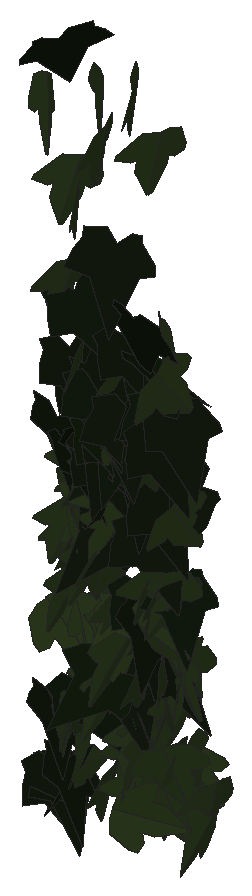
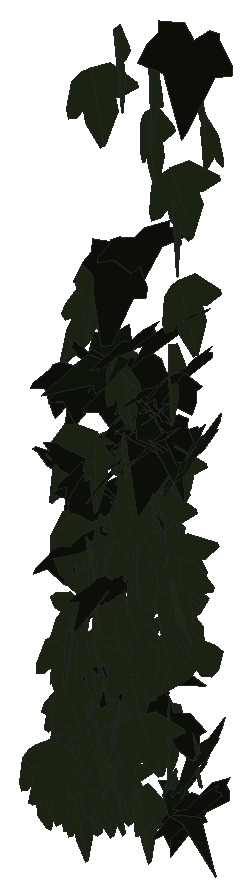
# SketchUp Ruby script. Lengths in inches.
U = 1.inch
M = Sketchup.active_model
def pt(a) = Geom::Point3d.new(a.map { |v| v * U })
def face(e, loops, mat)
  f = e.add_face(loops[0].map { |a| pt(a) })
  loops[1..].each { |l| e.add_face(l.map { |a| pt(a) }).erase! }
  f.material = f.back_material = mat if mat
  f
end
# faces: each face lists its corners as indices into pts; further lists are holes
def faces(e, pts, list, mat = nil) = list.each { |f| face(e, (f[0].is_a?(Array) ? f : [f]).map { |l| l.map { |i| pts[i] } }, mat) }
# xy, xz, yz: faces in a plane at the given z, y or x. An outline is a flat list of corners, or four numbers for a rectangle; further outlines are holes
def ring(l) = l.size == 4 ? [[l[0], l[1]], [l[2], l[1]], [l[2], l[3]], [l[0], l[3]]] : l.each_slice(2).to_a
def flat(e, list, mat, &to3) = list.each { |f| face(e, (f[0].is_a?(Array) ? f : [f]).map { |l| ring(l).map { |u, v| to3.(u, v) } }, mat) }
def xy(e, z, list, mat = nil) = flat(e, list, mat) { |x, y| [x, y, z] }
def xz(e, y, list, mat = nil) = flat(e, list, mat) { |x, z| [x, y, z] }
def yz(e, x, list, mat = nil) = flat(e, list, mat) { |y, z| [x, y, z] }
def lines(e, pts, list) = list.each { |a, b| e.add_line(pt(pts[a]), pt(pts[b])) }
# prism: a flat outline (further loops are holes) pulled along v
def prism(e, loops, v, mat = nil)
  f = face(e, loops, mat); d = Geom::Vector3d.new(v.map { |x| x * U })
  f.pushpull(f.normal.samedirection?(d) ? d.length : -d.length)
end
def box(e, o, s, mat = nil) = prism(e, [[o, [o[0] + s[0], o[1], o[2]], [o[0] + s[0], o[1] + s[1], o[2]], [o[0], o[1] + s[1], o[2]]]], [0, 0, s[2]], mat)
def at(x, y, z, deg = 0) = Geom::Transformation.translation(pt([x, y, z])) * Geom::Transformation.rotation(ORIGIN, Z_AXIS, deg.degrees)
def axes(o, x, y, z) = Geom::Transformation.new([*x, 0, *y, 0, *z, 0, *pt(o).to_a, 1])
def part(name) = M.definitions.add(name)
# library, detail: a bought-in or finely detailed component or shape, given as its bounding box
def library(name, o, s) = part(name).tap { |d| box(d.entities, o, s) }
def detail(e, o, s) = box(e.add_group.entities, o, s)
def put(e, d, t, mat = nil) = e.add_instance(d, t).tap { |i| i.material = mat if mat }
def group(e, t, mat = nil) = e.add_group.tap { |g| g.transformation = t; g.material = mat if mat }.entities
root = M.entities
M.materials.add("efeu1").color = [18, 25, 13]
M.materials.add("efeu2").color = [43, 57, 29]
c1 = part("ivyleaf_9")
p = [[1.54,2.16,1.25],[1.36,2.04,1.19],[-0.21,0.99,0.68],[-0.71,1.11,0.82],[-0.85,0.86,0.67],[-0.8,0.17,0.21],
  [-0.9,-0.01,0.1],[-0.67,-0.16,-0.02],[-0.08,-0.08,-0.05],[-0.03,-0.6,-0.4],[0.65,-0.88,-0.66],[0.83,-0.6,-0.49],
  [1.29,-0.42,-0.43],[1.8125,-0.07,-0.26],[1.21,0.44,0.15]]
faces(c1.entities,p,[[0,1,2,3,4,5,6,7,8,9,10,11,12,13,14]],"efeu1")
c2 = part("ivyleaf_10")
p = [[0,0.5,-0.03],[-0.0625,2.02,-0.43],[-0.19,2.01,-0.46],[-0.54,1.05,-0.29],[-0.52,0.625,-0.18],[-0.83,0.76,-0.28],
  [-1.16,0.64,-0.33],[-1.15,0.33,-0.24],[-0.77,-0.39,0.02],[-0.3,-0.51,0.16],[0.04,-0.48,0.23],[-0.02,2.01,-0.4375],
  [-0.06,2.01,-0.43],[0.04,-0.49,0.23],[0.67,-0.49,0.14],[1.38,0.36,-0.2],[1.375,0.51,-0.24],[0.81,0.65,-0.19],
  [0.62,0.59,-0.15],[0.6,1.09,-0.28],[0.5,1.23,-0.31]]
faces(c2.entities,p,[[0,1,2,3,4,5,6,7,8,9,10],[11,12,0,13,14,15,16,17,18,19,20]],"efeu2")
put(root,c1,axes([512.25,136.02,185.85],[0.17121,-0.66389,0.41643],[0.14297,-0.39264,-0.68474],[0.77053,0.22037,0.03452]))
put(root,c2,axes([512.8,136.1,191.76],[-0.23988,-0.65077,0.29698],[-0.05706,-0.29483,-0.69214],[0.71305,-0.24252,0.04452]))
put(root,c2,axes([512.39,135.42,204.18],[0.63102,-0.41173,0.31313],[0.32609,-0.06679,-0.74496],[0.40155,0.70127,0.11289]))
put(root,c2,axes([512.73,136.19,190.89],[0.29316,-0.70256,0.01967],[0.00631,-0.01868,-0.76127],[0.70281,0.29322,-0.00137]))
put(root,c1,axes([513.13,135.59,184.39],[-0.43077,0.62259,0.10496],[-0.07146,0.07817,-0.75695],[-0.62732,-0.43643,0.01415]))
put(root,c2,axes([512.82,136.26,191.31],[-0.52598,-0.52412,-0.07313],[0.07237,0.03089,-0.74197],[0.52422,-0.53014,0.02906]))
put(root,c2,axes([512.87,136.08,189.88],[0.00273,-0.64219,0.39214],[0.02346,-0.39188,-0.64193],[0.75209,0.01456,0.0186]))
put(root,c1,axes([512.58,135.55,184.57],[0.11322,-0.65761,-0.38062],[-0.08148,0.3721,-0.66712],[0.75544,0.1387,-0.01491]))
put(root,c1,axes([512.63,135.93,184.36],[0.09548,-0.75103,-0.16729],[-0.02977,0.16484,-0.75703],[0.76886,0.09965,-0.00854]))
put(root,c2,axes([513,135.64,199.0625],[-0.11608,-0.78207,0.08337],[-0.01662,-0.08182,-0.79062],[0.78632,-0.11718,-0.0044]))
put(root,c2,axes([512.55,135.68,188.94],[0.43104,0.49262,0.46939],[0.30894,0.35339,-0.65457],[-0.60626,0.53032,0.00017]))
put(root,c1,axes([512.62,135.67,194.54],[0.19979,-0.68286,0.34135],[0.14695,-0.31185,-0.70986],[0.74915,0.24328,0.04821]))
put(root,c2,axes([513.19,135.29,186.32],[0.52518,-0.53151,-0.21282],[-0.13994,0.16087,-0.74709],[0.55517,0.54335,0.01301]))
put(root,c1,axes([513.22,135,206.06],[0.26904,0.77907,-0.13785],[-0.0424,-0.1312,-0.82421],[-0.79003,0.27235,-0.00271]))
put(root,c2,axes([513.16,135.91,184.79],[0.16834,-0.33193,-0.63703],[0.04962,0.6581,-0.32979],[0.7166,0.0324,0.17249]))
put(root,c2,axes([513.35,136.875,186.88],[-0.5621,-0.38238,0.26694],[-0.08089,-0.33178,-0.6456],[0.45926,-0.52643,0.213]))
put(root,c2,axes([513.35,135.53,202.18],[-0.32855,-0.70465,0.21746],[-0.00138,-0.23747,-0.7716],[0.73744,-0.31439,0.09544]))
put(root,c2,axes([513.24,135.64,201.43],[0.46456,-0.6346,-0.16218],[0.02329,0.21472,-0.77343],[0.65459,0.44274,0.14262]))
put(root,c2,axes([513.84,135.73,191.36],[-0.22843,0.05655,0.74398],[-0.74006,-0.11613,-0.2184],[0.0949,-0.76954,0.08763]))
put(root,c2,axes([513.37,135.58,186.62],[0.19506,-0.62436,-0.44065],[-0.0684,0.43869,-0.65186],[0.76113,0.19943,0.05435]))
put(root,c2,axes([513.39,136.28,192.96],[-0.29712,-0.70174,0.08196],[-0.02507,-0.07839,-0.76201],[0.70607,-0.29808,0.00743]))
put(root,c2,axes([513.16,136.48,188.93],[0.30224,0.67377,0.01159],[0.00109,0.01222,-0.73844],[-0.67386,0.30222,0.00401]))
put(root,c1,axes([512.93,135.6875,184.65],[0.26823,-0.71704,0.18582],[0.04112,-0.18291,-0.76517],[0.73959,0.27022,-0.02485]))
put(root,c2,axes([513.28,136.06,192.25],[0.17181,0.63478,0.40598],[-0.04092,0.42365,-0.64508],[-0.75239,0.12191,0.12779]))
put(root,c2,axes([513.4,136.04,191.22],[-0.44298,0.6305,0.26282],[0.11574,-0.23944,0.76949],[0.67321,0.45604,0.04065]))
put(root,c2,axes([513.47,135.5,196.96],[0.28545,-0.66525,-0.30561],[-0.04253,0.3124,-0.71975],[0.73086,0.278,0.07748]))
put(root,c2,axes([513.48,135.84,193.11],[0.14567,-0.76213,-0.00746],[-0.00245,0.00712,-0.77593],[0.76217,0.14568,-0.00107]))
put(root,c1,axes([513.14,135.54,196.76],[0.19066,-0.74802,-0.1562],[-0.0054,0.15966,-0.77121],[0.76414,0.18776,0.03352]))
put(root,c1,axes([513.09,135.84,198.26],[0.2356,-0.67759,-0.31851],[0.08286,0.35545,-0.69489],[0.74412,0.17495,0.17822]))
put(root,c2,axes([513.7,135.63,193.89],[-0.52211,-0.50137,0.25286],[-0.09213,-0.2641,-0.71391],[0.55391,-0.51651,0.11959]))
put(root,c2,axes([513.66,135.96,190.96],[-0.11803,-0.65996,0.36858],[-0.02879,-0.36885,-0.66966],[0.75536,-0.11718,0.03207]))
put(root,c1,axes([513.2,135.33,194.15],[0.50606,-0.58909,0.01522],[0.00808,-0.01313,-0.77661],[0.58923,0.50612,-0.00243]))
put(root,c1,axes([513.2,135.91,186.97],[-0.13591,-0.25755,-0.75391],[0.55722,0.51589,-0.27669],[0.56941,-0.56632,0.09082]))
put(root,c2,axes([513.76,136.35,184.31],[0.17597,-0.72027,-0.09053],[-0.01826,0.08873,-0.74145],[0.72571,0.17688,0.0033]))
put(root,c1,axes([514.12,135.24,195.02],[-0.32198,0.72176,0.01967],[-0.00865,0.01767,-0.79032],[-0.72197,-0.32209,0.0007]))
put(root,c1,axes([513.93,135.43,194.88],[0.3543,0.74278,-0.06207],[-0.03684,-0.05119,-0.82287],[-0.74446,0.35603,0.01119]))
put(root,c2,axes([514.02,136.53,188.28],[-0.2659,-0.69247,0.08325],[-0.02154,-0.0809,-0.74171],[0.69712,-0.26662,0.00884]))
put(root,c2,axes([514.41,136.86,184.91],[-0.27999,0.21572,0.6234],[-0.58852,0.22425,-0.34193],[-0.298,-0.64555,0.08954]))
put(root,c2,axes([514.15,136.04,193.51],[-0.1752,-0.75203,0.11088],[-0.01439,-0.11049,-0.77209],[0.76002,-0.17545,0.01094]))
put(root,c2,axes([514.26,135.87,191.35],[-0.57986,-0.45419,0.14176],[-0.10103,-0.10084,-0.73637],[0.46494,-0.58835,0.01678]))
put(root,c2,axes([514.18,135.55,191.25],[0.08005,-0.75655,-0.10705],[-0.00412,0.1072,-0.76074],[0.76408,0.07984,0.00711]))
put(root,c2,axes([513.6875,135.08,193.375],[0.01712,-0.22317,0.76558],[0.45523,0.63146,0.17389],[-0.65474,0.43321,0.14093]))
put(root,c1,axes([513.7,135.53,196.51],[-0.13786,-0.34361,-0.6958],[0.46042,0.53265,-0.35426],[0.62467,-0.46843,0.10756]))
put(root,c2,axes([514.16,135.9,187.23],[-0.03601,-0.55699,0.49682],[0.10069,-0.49647,-0.54931],[0.73954,0.04047,0.09898]))
put(root,c1,axes([514.4,135.74,187.78],[-0.56306,-0.4476,0.28525],[-0.202,-0.20385,-0.7186],[0.49083,-0.59737,0.03149]))
put(root,c2,axes([514.21,136.24,189.62],[0.03679,-0.74511,0.13637],[0.03521,-0.1347,-0.74549],[0.75667,0.04249,0.02806]))
put(root,c2,axes([514.24,135.43,203.4375],[0.18275,-0.78477,-0.11098],[0.00147,0.11422,-0.80531],[0.79257,0.18073,0.02708]))
put(root,c1,axes([514.66,135.18,193.3],[-0.2741,0.59282,0.51746],[-0.22474,0.46615,-0.65309],[-0.75412,-0.3544,0.00655]))
put(root,c1,axes([514.03,136.02,194.24],[-0.08895,-0.74088,0.20839],[-0.01658,-0.20788,-0.74616],[0.76945,-0.09013,0.00801]))
put(root,c1,axes([513.95,135.58,194.28],[0.27097,-0.66444,-0.29611],[-0.02825,0.30614,-0.71279],[0.72689,0.25959,0.08268]))
put(root,c2,axes([514.28,135.29,204.91],[0.56963,-0.56149,-0.18704],[0.01429,0.27258,-0.77474],[0.59165,0.534,0.1988]))
put(root,c1,axes([514.59,135.61,192.25],[-0.81295,-0.15313,-0.03686],[0.03748,0.00013,-0.82722],[0.15298,-0.81379,0.0068]))
put(root,c1,axes([513.98,135.56,196.05],[0.12458,-0.77171,-0.14079],[0.10346,0.15748,-0.7716],[0.77759,0.10269,0.12522]))
put(root,c2,axes([514.37,136.06,194.59],[0.20582,-0.74294,0.04333],[0.05377,-0.03,-0.76968],[0.74226,0.20819,0.04374]))
put(root,c1,axes([514.67,136.08,194.47],[-0.7419,-0.19795,0.05758],[-0.0545,-0.01909,-0.76784],[0.19883,-0.74389,0.00438]))
put(root,c2,axes([514.4,135.78,191.11],[0.12669,-0.69615,-0.24596],[0.0853,0.26168,-0.69672],[0.73338,0.08983,0.12353]))
put(root,c2,axes([514.5,136.94,185.91],[0.21403,-0.68514,0.11083],[0.01362,-0.11181,-0.71751],[0.69391,0.21352,-0.0201]))
put(root,c2,axes([514.48,135.76,188.45],[0.00445,-0.57781,0.48339],[0.10521,-0.47819,-0.57256],[0.74597,0.07089,0.07787]))
put(root,c2,axes([514.57,136.14,196.52],[-0.01684,-0.77554,0.00348],[-0.00083,-0.00347,-0.77572],[0.77555,-0.01685,-0.00076]))
put(root,c2,axes([514.6,136.55,185.46],[-0.29293,-0.65264,0.18639],[0.00575,-0.20539,-0.71012],[0.67871,-0.27994,0.08646]))
put(root,c2,axes([514.67,135.66,192.41],[-0.24468,-0.60599,0.41848],[-0.06904,-0.42016,-0.64878],[0.7332,-0.24179,0.07857]))
put(root,c2,axes([514.35,135.8,188.2],[0.28379,0.33168,-0.70111],[0.34152,0.61686,0.43006],[0.69637,-0.4377,0.07481]))
put(root,c1,axes([514.24,135.66,194.93],[0.31041,-0.69709,-0.19095],[0.0485,0.22743,-0.75145],[0.72114,0.28476,0.13273]))
put(root,c1,axes([514.29,135.41,195.13],[0.22789,-0.68741,-0.30167],[0.02736,0.32266,-0.71457],[0.75019,0.19705,0.1177]))
put(root,c2,axes([514.55,136.49,185.25],[-0.17048,0.66531,-0.22893],[0.06062,-0.22079,-0.68679],[-0.70098,-0.1809,-0.00372]))
put(root,c1,axes([514.53,135.67,200.21],[-0.25262,-0.74161,-0.16443],[0.04273,0.15913,-0.78339],[0.75842,-0.25599,-0.01063]))
put(root,c1,axes([515.03,135.67,195.92],[-0.75708,0.20191,-0.12469],[0.11088,-0.06762,-0.7827],[-0.20981,-0.76429,0.03631]))
put(root,c2,axes([514.74,136.13,186.375],[-0.45154,0.56141,0.074],[-0.05217,0.05299,-0.72043],[-0.56386,-0.45448,0.0074]))
put(root,c2,axes([514.82,136.76,184.71],[-0.07405,-0.71007,0.10685],[-0.00795,-0.1066,-0.71392],[0.71802,-0.07441,0.00311]))
put(root,c2,axes([514.69,135.63,194.9],[0.05471,0.76286,-0.02279],[-0.00098,-0.02278,-0.76482],[-0.7632,0.05471,-0.00065]))
put(root,c1,axes([514.46,136.0625,197.37],[0.26223,-0.67127,-0.29909],[-0.00477,0.316,-0.71341],[0.73487,0.24158,0.10209]))
put(root,c1,axes([514.5625,136.08,187.79],[-0.26325,-0.56288,-0.47031],[0.22757,0.41236,-0.62089],[0.69731,-0.34707,0.02507]))
put(root,c2,axes([514.96,136.08,184.59],[-0.35461,-0.56352,0.25401],[-0.0609,-0.25957,-0.66086],[0.61512,-0.35056,0.081]))
put(root,c2,axes([514.85,136.18,186.51],[-0.50662,0.51359,0.07012],[-0.0453,0.05381,-0.72139],[-0.51637,-0.50861,-0.00551]))
put(root,c2,axes([514.99,136.18,186.09],[-0.30301,-0.61327,0.24037],[0.01921,-0.2727,-0.67153],[0.65841,-0.27428,0.13021]))
put(root,c1,axes([514.91,135.54,195.29],[-0.63043,-0.30698,-0.31151],[0.26678,0.16312,-0.70067],[0.34656,-0.68401,-0.02729]))
put(root,c2,axes([515.08,136.52,186.12],[-0.16485,-0.63964,0.30856],[-0.04113,-0.30763,-0.65969],[0.70898,-0.16657,0.03347]))
put(root,c2,axes([514.92,136.78,185.83],[-0.25761,0.67358,0.02736],[-0.01828,0.0223,-0.7211],[-0.67389,-0.2581,0.0091]))
put(root,c2,axes([515.03,136.42,189.125],[0.19949,-0.73235,-0.03365],[-0.00729,0.03289,-0.75903],[0.73308,0.19962,0.00161]))
put(root,c2,axes([514.92,136.27,185.66],[0.19958,-0.57233,0.42674],[0.15986,-0.39602,-0.6059],[0.69578,0.25516,0.0168]))
put(root,c1,axes([514.95,135.58,195.6],[-0.17756,-0.71373,-0.27923],[0.06089,0.27258,-0.73546],[0.76398,-0.18761,-0.00628]))
put(root,c2,axes([515.28,135.84,188.11],[0.13523,-0.7155,-0.24789],[-0.03584,0.24548,-0.72811],[0.75638,0.13956,0.00982]))
put(root,c2,axes([515.28,137.02,185.21],[0.04805,-0.71284,0.10847],[-0.00929,-0.10932,-0.71427],[0.72099,0.0461,-0.01643]))
put(root,c2,axes([515.29,136.6,188.43],[0.06313,-0.75009,-0.02448],[0.00213,0.02474,-0.75273],[0.75048,0.06302,0.0042]))
put(root,c1,axes([514.95,136.125,193.52],[0.11935,-0.70852,0.26439],[0.01619,-0.26521,-0.71802],[0.75607,0.11752,-0.02636]))
put(root,c2,axes([515.32,137.02,184.04],[0.09741,-0.72191,-0.0235],[-0.01013,0.02234,-0.72842],[0.72223,0.09768,-0.00705]))
put(root,c1,axes([514.95,136.15,190.29],[0.12341,-0.63823,-0.40495],[0.03462,0.41465,-0.64298],[0.75507,0.0853,0.09567]))
put(root,c1,axes([514.83,136.13,196.92],[0.72541,-0.27976,-0.0358],[0.06417,0.25992,-0.73081],[0.27465,0.67819,0.26532]))
put(root,c2,axes([515.49,136.99,184.38],[-0.36892,-0.51319,0.36236],[-0.09128,-0.37197,-0.61974],[0.62156,-0.35923,0.12406]))
put(root,c2,axes([515.4,136.15,193.9375],[0.12244,-0.73575,-0.17778],[0.04193,0.18641,-0.74258],[0.75576,0.10885,0.07]))
put(root,c2,axes([515.42,135.25,205.34],[0.40712,-0.68811,-0.19455],[-0.0132,0.2166,-0.79373],[0.71497,0.39583,0.09612]))
put(root,c2,axes([515.05,135.49,184.02],[0.15911,0.18928,0.74365],[0.36719,0.64809,-0.24353],[-0.6738,0.39788,0.0429]))
put(root,c1,axes([515.67,136.02,196.58],[-0.70887,-0.15793,-0.29073],[0.29845,-0.00854,-0.72306],[0.1428,-0.76612,0.068]))
put(root,c1,axes([515.67,134.98,198.77],[0.6484,0.20638,-0.50511],[-0.4812,-0.15359,-0.68045],[-0.25726,0.80745,-0.00033]))
put(root,c2,axes([515.7,136.9,186.9375],[-0.09942,-0.68694,0.23503],[0.00931,-0.23841,-0.69288],[0.72597,-0.09102,0.04107]))
put(root,c2,axes([515.84,136.04,187.16],[0.20397,-0.51904,-0.48633],[-0.19774,0.44461,-0.55745],[0.68324,0.28363,-0.01615]))
put(root,c2,axes([515.72,136.29,184.46],[-0.54941,-0.48068,-0.18892],[0.15985,0.10402,-0.72954],[0.49111,-0.57159,0.02611]))
put(root,c1,axes([515.44,135.75,189.58],[0.09826,-0.67145,0.35087],[0.02967,-0.35013,-0.67833],[0.75701,0.10088,-0.01896]))
put(root,c2,axes([515.84,135.375,191.12],[0.16545,-0.61795,-0.45472],[-0.0302,0.45957,-0.63552],[0.76663,0.15146,0.07309]))
put(root,c2,axes([515.92,135.66,190.76],[0.3464,-0.69048,0.02761],[0.00285,-0.02945,-0.77243],[0.69103,0.34625,-0.01066]))
put(root,c2,axes([516.02,136.6875,188.26],[-0.31268,-0.66254,-0.06306],[0.07511,0.0341,-0.73068],[0.66128,-0.31714,0.05317]))
put(root,c1,axes([515.76,135.99,195.84],[-0.05443,-0.73111,-0.26218],[0.04228,0.25965,-0.73282],[0.77555,-0.06547,0.02155]))
put(root,c1,axes([515.73,135.83,193.35],[0.1533,-0.69187,-0.32191],[-0.02486,0.32364,-0.70743],[0.76269,0.14961,0.04164]))
put(root,c1,axes([515.74,135.57,192.54],[-0.19304,-0.58333,-0.50813],[0.22139,0.46015,-0.61236],[0.74125,-0.28935,0.05057]))
put(root,c2,axes([515.84,137,185.14],[-0.58423,-0.24718,-0.35629],[0.35253,0.07738,-0.63175],[0.25252,-0.67991,0.05763]))
put(root,c2,axes([516.03,135.72,198.23],[-0.58126,0.51723,-0.15152],[-0.00783,-0.23093,-0.75826],[-0.53891,-0.55452,0.17445]))
put(root,c2,axes([516.16,135.32,203.99],[-0.30101,-0.75399,0.07161],[-0.0151,-0.07107,-0.81176],[0.75723,-0.30114,0.01227]))
put(root,c2,axes([515.52,135.47,189.7],[-0.24027,0.08563,-0.74359],[0.71724,-0.19703,-0.25444],[-0.21408,-0.7562,-0.01791]))
put(root,c2,axes([516.5,135.54,187.46],[0.32196,-0.11346,0.72174],[-0.67197,0.2636,0.34119],[-0.28678,-0.74504,0.01081]))
put(root,c2,axes([516.3,135.37,191.21],[-0.65097,-0.54586,0.01318],[-0.00988,-0.00873,-0.84954],[0.54593,-0.65104,0.00034]))
put(root,c1,axes([516.58,136.45,193.59],[-0.74837,-0.07417,0.10492],[-0.10285,-0.02579,-0.75187],[0.077,-0.75524,0.01537]))
put(root,c2,axes([516.35,135.99,188.26],[0.30155,-0.49517,-0.51072],[-0.09947,0.51991,-0.56281],[0.70436,0.28541,0.13917]))
put(root,c2,axes([516.37,136.2,188.5625],[-0.26854,0.59943,0.34639],[-0.18677,0.29504,-0.65535],[-0.66665,-0.32412,0.04407]))
put(root,c1,axes([515.99,135.83,188.7],[0.43238,-0.58718,-0.2582],[-0.06967,0.26656,-0.72284],[0.63765,0.42729,0.09611]))
put(root,c2,axes([516.48,135.9,190.92],[-0.0808,-0.60541,0.47373],[-0.05975,-0.46995,-0.61078],[0.7664,-0.10046,0.00232]))
put(root,c1,axes([516.12,135.26,195.54],[0.18525,-0.66908,-0.41049],[-0.10924,0.39569,-0.69426],[0.77733,0.21506,0.00026]))
put(root,c2,axes([516.37,135.51,186.11],[-0.63312,-0.44401,-0.19405],[0.15879,0.11154,-0.77329],[0.4578,-0.65272,-0.00015]))
put(root,c2,axes([516.48,136.14,186.07],[-0.03464,-0.66941,-0.28687],[0.07196,0.28264,-0.66823],[0.72472,-0.06006,0.05264]))
put(root,c1,axes([516.24,136.14,190.85],[-0.05042,-0.75448,-0.14466],[0.02452,0.14332,-0.75602],[0.76783,-0.05412,0.01464]))
put(root,c2,axes([516.51,135,189.12],[0.39272,-0.53614,-0.38819],[-0.023,0.44005,-0.63103],[0.66153,0.33359,0.20851]))
put(root,c2,axes([516.56,134.95,197.375],[-0.13116,-0.67818,-0.52389],[0.19724,0.49187,-0.68611],[0.83395,-0.22299,0.07988]))
put(root,c2,axes([516.37,135.83,188.66],[-0.54116,0.26785,-0.43791],[0.36617,-0.24453,-0.60207],[-0.35977,-0.65179,0.04592]))
put(root,c1,axes([516.41,135.86,195.89],[-0.0895,-0.69705,-0.33683],[0.0706,0.33031,-0.70232],[0.77094,-0.11117,0.02521]))
put(root,c2,axes([516.8,136.72,184.72],[-0.12444,-0.71897,0.0291],[-0.00486,-0.02869,-0.72965],[0.71954,-0.12453,0.0001]))
put(root,c2,axes([516.72,135.34,193.4],[-0.22642,-0.64247,-0.42657],[0.17166,0.39143,-0.68067],[0.75184,-0.28286,0.02695]))
put(root,c2,axes([516.63,136.67,183.77],[0.05956,-0.3801,0.62989],[0.24645,-0.58513,-0.37639],[0.69318,0.2407,0.0797]))
